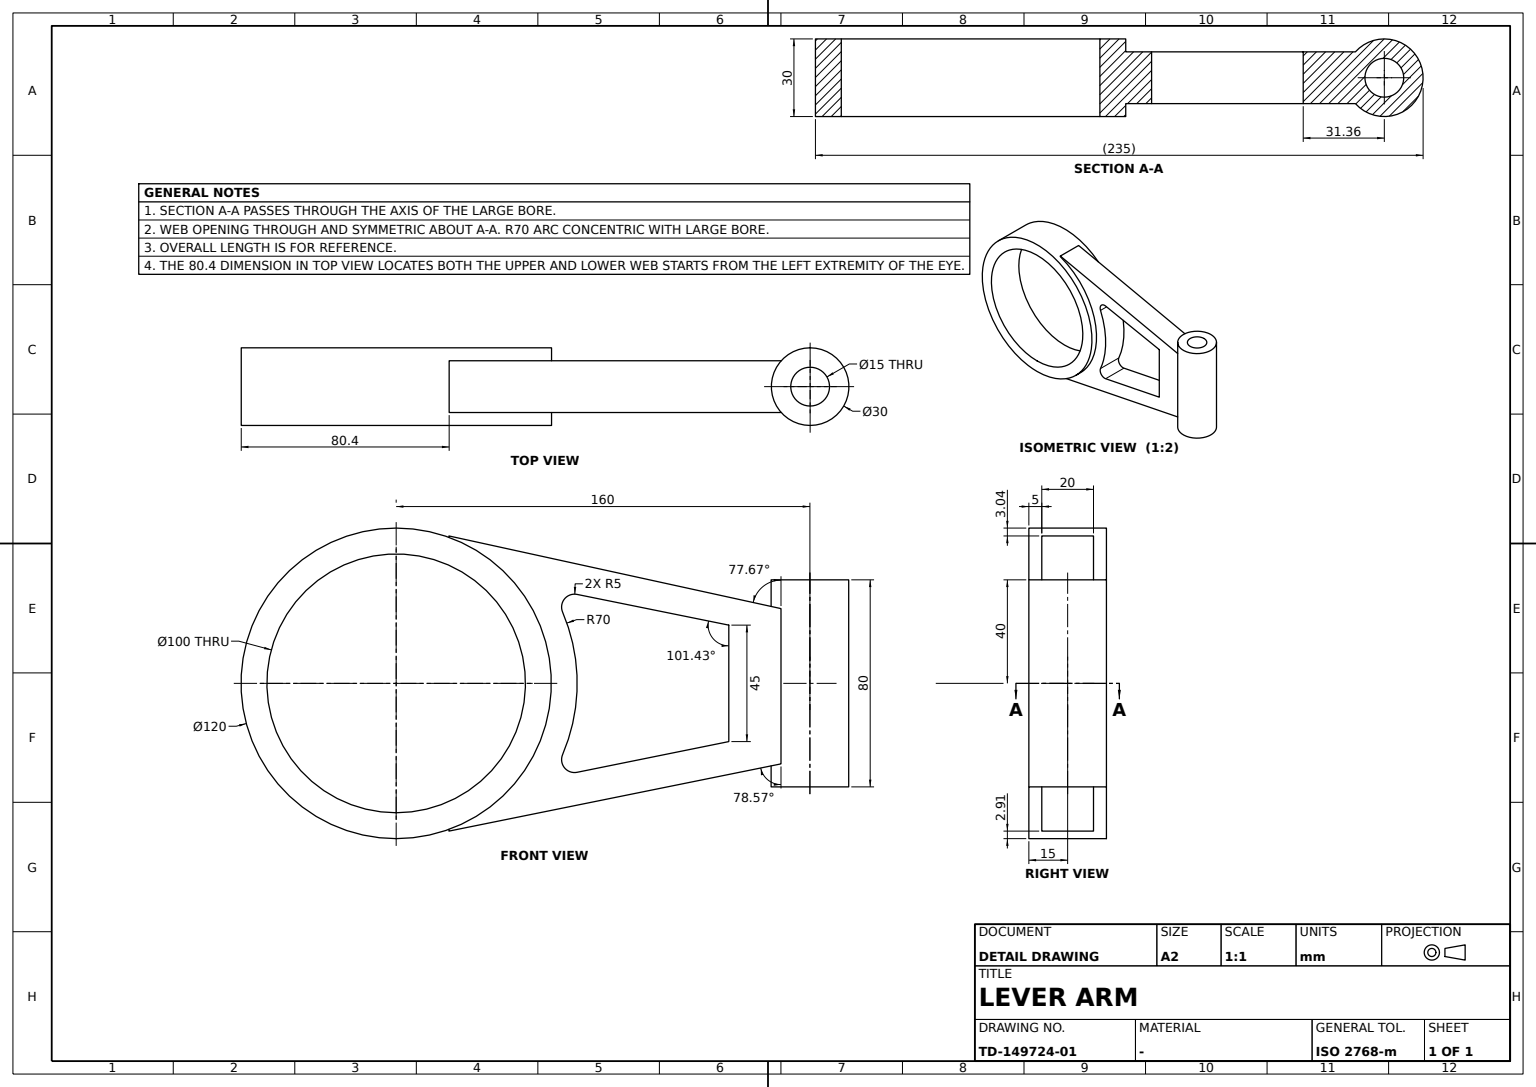
ISO-10303-21;
HEADER;
FILE_DESCRIPTION((''),'2;1');
FILE_NAME('','',(''),(''),'','','');
FILE_SCHEMA(('AUTOMOTIVE_DESIGN'));
ENDSEC;
DATA;
#1=APPLICATION_CONTEXT('');
#2=PRODUCT_CONTEXT('',#1,'mechanical');
#3=PRODUCT('','','',(#2));
#4=PRODUCT_DEFINITION_FORMATION('','',#3);
#5=PRODUCT_DEFINITION_CONTEXT('',#1,'design');
#6=PRODUCT_DEFINITION('','',#4,#5);
#7=PRODUCT_DEFINITION_SHAPE('','',#6);
#8=(LENGTH_UNIT()NAMED_UNIT(*)SI_UNIT(.MILLI.,.METRE.));
#9=(NAMED_UNIT(*)PLANE_ANGLE_UNIT()SI_UNIT($,.RADIAN.));
#10=(NAMED_UNIT(*)SI_UNIT($,.STERADIAN.)SOLID_ANGLE_UNIT());
#11=UNCERTAINTY_MEASURE_WITH_UNIT(LENGTH_MEASURE(0.005),#8,'distance_accuracy_value','');
#12=(GEOMETRIC_REPRESENTATION_CONTEXT(3)GLOBAL_UNCERTAINTY_ASSIGNED_CONTEXT((#11))GLOBAL_UNIT_ASSIGNED_CONTEXT((#8,#9,#10))REPRESENTATION_CONTEXT('',''));
#13=CARTESIAN_POINT('',(22.5,128.637224,-10.));
#14=VERTEX_POINT('',#13);
#15=CARTESIAN_POINT('',(34.367829,69.959986,-10.));
#16=VERTEX_POINT('',#15);
#17=DIRECTION('',(0.198241947,-0.980153116,0.));
#18=VECTOR('',#17,1000.);
#19=LINE('',#13,#18);
#20=EDGE_CURVE('',#14,#16,#19,.T.);
#21=ORIENTED_EDGE('',*,*,#20,.T.);
#22=CARTESIAN_POINT('',(34.367829,69.959986,10.));
#23=VERTEX_POINT('',#22);
#24=DIRECTION('',(0.,0.,1.));
#25=VECTOR('',#24,1000.);
#26=LINE('',#15,#25);
#27=EDGE_CURVE('',#23,#16,#26,.F.);
#28=ORIENTED_EDGE('',*,*,#27,.F.);
#29=CARTESIAN_POINT('',(22.5,128.637224,10.));
#30=VERTEX_POINT('',#29);
#31=CARTESIAN_POINT('',(42.646309,29.029308,10.));
#32=LINE('',#31,#18);
#33=EDGE_CURVE('',#30,#23,#32,.T.);
#34=ORIENTED_EDGE('',*,*,#33,.F.);
#35=DIRECTION('',(0.,0.,-1.));
#36=VECTOR('',#35,1000.);
#37=LINE('',#29,#36);
#38=EDGE_CURVE('',#30,#14,#37,.T.);
#39=ORIENTED_EDGE('',*,*,#38,.T.);
#40=EDGE_LOOP('',(#21,#28,#34,#39));
#41=FACE_BOUND('',#40,.T.);
#42=DIRECTION('',(0.980153116,0.198241947,0.));
#43=AXIS2_PLACEMENT_3D('',#29,#42,#17);
#44=PLANE('',#43);
#45=ADVANCED_FACE('',(#41),#44,.F.);
#46=CARTESIAN_POINT('',(56.424141,20.403831,-10.));
#47=VERTEX_POINT('',#46);
#48=CARTESIAN_POINT('',(56.424141,20.403831,10.));
#49=VERTEX_POINT('',#48);
#50=LINE('',#48,#25);
#51=EDGE_CURVE('',#47,#49,#50,.T.);
#52=ORIENTED_EDGE('',*,*,#51,.F.);
#53=CARTESIAN_POINT('',(57.088126,20.403831,-10.));
#54=VERTEX_POINT('',#53);
#55=CARTESIAN_POINT('',(0.,20.403831,-10.));
#56=DIRECTION('',(1.,0.,0.));
#57=VECTOR('',#56,1000.);
#58=LINE('',#55,#57);
#59=EDGE_CURVE('',#47,#54,#58,.T.);
#60=ORIENTED_EDGE('',*,*,#59,.T.);
#61=CARTESIAN_POINT('',(57.088126,20.403831,10.));
#62=VERTEX_POINT('',#61);
#63=LINE('',#61,#36);
#64=EDGE_CURVE('',#62,#54,#63,.T.);
#65=ORIENTED_EDGE('',*,*,#64,.F.);
#66=CARTESIAN_POINT('',(0.,20.403831,10.));
#67=LINE('',#66,#57);
#68=EDGE_CURVE('',#49,#62,#67,.T.);
#69=ORIENTED_EDGE('',*,*,#68,.F.);
#70=EDGE_LOOP('',(#52,#60,#65,#69));
#71=FACE_BOUND('',#70,.T.);
#72=DIRECTION('',(0.,-1.,0.));
#73=AXIS2_PLACEMENT_3D('',#66,#72,#35);
#74=PLANE('',#73);
#75=ADVANCED_FACE('',(#71),#74,.T.);
#76=CARTESIAN_POINT('',(-40.,160.,-15.));
#77=VERTEX_POINT('',#76);
#78=CARTESIAN_POINT('',(-40.,160.,0.));
#79=AXIS2_PLACEMENT_3D('',#78,#56,#35);
#80=CIRCLE('',#79,15.);
#81=EDGE_CURVE('',#77,#77,#80,.T.);
#82=ORIENTED_EDGE('',*,*,#81,.F.);
#83=EDGE_LOOP('',(#82));
#84=FACE_BOUND('',#83,.T.);
#85=CARTESIAN_POINT('',(-40.,160.,-7.5));
#86=VERTEX_POINT('',#85);
#87=CIRCLE('',#79,7.5);
#88=EDGE_CURVE('',#86,#86,#87,.T.);
#89=ORIENTED_EDGE('',*,*,#88,.T.);
#90=EDGE_LOOP('',(#89));
#91=FACE_BOUND('',#90,.T.);
#92=CARTESIAN_POINT('',(-40.,0.,0.));
#93=DIRECTION('',(0.,1.,0.));
#94=AXIS2_PLACEMENT_3D('',#92,#56,#93);
#95=PLANE('',#94);
#96=ADVANCED_FACE('',(#84,#91),#95,.F.);
#97=CARTESIAN_POINT('',(40.,160.,-7.5));
#98=VERTEX_POINT('',#97);
#99=CARTESIAN_POINT('',(40.,160.,0.));
#100=AXIS2_PLACEMENT_3D('',#99,#56,#35);
#101=CIRCLE('',#100,7.5);
#102=EDGE_CURVE('',#98,#98,#101,.T.);
#103=ORIENTED_EDGE('',*,*,#102,.T.);
#104=EDGE_LOOP('',(#103));
#105=FACE_BOUND('',#104,.T.);
#106=ORIENTED_EDGE('',*,*,#88,.F.);
#107=EDGE_LOOP('',(#106));
#108=FACE_BOUND('',#107,.T.);
#109=CARTESIAN_POINT('',(0.,160.,0.));
#110=AXIS2_PLACEMENT_3D('',#109,#56,#93);
#111=CYLINDRICAL_SURFACE('',#110,7.5);
#112=ADVANCED_FACE('',(#105,#108),#111,.F.);
#113=CARTESIAN_POINT('',(-34.367829,69.959986,10.));
#114=VERTEX_POINT('',#113);
#115=CARTESIAN_POINT('',(-34.367829,69.959986,-10.));
#116=VERTEX_POINT('',#115);
#117=LINE('',#115,#25);
#118=EDGE_CURVE('',#114,#116,#117,.F.);
#119=ORIENTED_EDGE('',*,*,#118,.F.);
#120=CARTESIAN_POINT('',(-27.502593,64.370858,10.));
#121=VERTEX_POINT('',#120);
#122=CARTESIAN_POINT('',(-29.467064,68.968777,10.));
#123=DIRECTION('',(-1.,0.,0.));
#124=AXIS2_PLACEMENT_3D('',#122,#35,#123);
#125=CIRCLE('',#124,5.);
#126=EDGE_CURVE('',#114,#121,#125,.F.);
#127=ORIENTED_EDGE('',*,*,#126,.T.);
#128=CARTESIAN_POINT('',(-27.502593,64.370858,-10.));
#129=VERTEX_POINT('',#128);
#130=CARTESIAN_POINT('',(-27.502593,64.370858,0.));
#131=LINE('',#130,#25);
#132=EDGE_CURVE('',#121,#129,#131,.F.);
#133=ORIENTED_EDGE('',*,*,#132,.T.);
#134=CARTESIAN_POINT('',(-29.467064,68.968777,-10.));
#135=AXIS2_PLACEMENT_3D('',#134,#24,#56);
#136=CIRCLE('',#135,5.);
#137=EDGE_CURVE('',#116,#129,#136,.T.);
#138=ORIENTED_EDGE('',*,*,#137,.F.);
#139=EDGE_LOOP('',(#119,#127,#133,#138));
#140=FACE_BOUND('',#139,.T.);
#141=CYLINDRICAL_SURFACE('',#135,5.);
#142=ADVANCED_FACE('',(#140),#141,.F.);
#143=CARTESIAN_POINT('',(50.,0.,-15.));
#144=VERTEX_POINT('',#143);
#145=CARTESIAN_POINT('',(0.,0.,-15.));
#146=AXIS2_PLACEMENT_3D('',#145,#24,#56);
#147=CIRCLE('',#146,50.);
#148=EDGE_CURVE('',#144,#144,#147,.T.);
#149=ORIENTED_EDGE('',*,*,#148,.T.);
#150=EDGE_LOOP('',(#149));
#151=FACE_BOUND('',#150,.T.);
#152=CARTESIAN_POINT('',(60.,0.,-15.));
#153=VERTEX_POINT('',#152);
#154=CIRCLE('',#146,60.);
#155=EDGE_CURVE('',#153,#153,#154,.T.);
#156=ORIENTED_EDGE('',*,*,#155,.F.);
#157=EDGE_LOOP('',(#156));
#158=FACE_BOUND('',#157,.T.);
#159=PLANE('',#146);
#160=ADVANCED_FACE('',(#151,#158),#159,.F.);
#161=CARTESIAN_POINT('',(-22.5,128.637224,10.));
#162=VERTEX_POINT('',#161);
#163=CARTESIAN_POINT('',(0.,128.637224,10.));
#164=LINE('',#163,#57);
#165=EDGE_CURVE('',#162,#30,#164,.T.);
#166=ORIENTED_EDGE('',*,*,#165,.T.);
#167=ORIENTED_EDGE('',*,*,#33,.T.);
#168=CARTESIAN_POINT('',(27.502593,64.370858,10.));
#169=VERTEX_POINT('',#168);
#170=CARTESIAN_POINT('',(29.467064,68.968777,10.));
#171=AXIS2_PLACEMENT_3D('',#170,#35,#123);
#172=CIRCLE('',#171,5.);
#173=EDGE_CURVE('',#169,#23,#172,.F.);
#174=ORIENTED_EDGE('',*,*,#173,.F.);
#175=CARTESIAN_POINT('',(0.,0.,10.));
#176=AXIS2_PLACEMENT_3D('',#175,#35,#123);
#177=CIRCLE('',#176,70.);
#178=EDGE_CURVE('',#169,#121,#177,.F.);
#179=ORIENTED_EDGE('',*,*,#178,.T.);
#180=ORIENTED_EDGE('',*,*,#126,.F.);
#181=CARTESIAN_POINT('',(-42.646309,29.029308,10.));
#182=DIRECTION('',(-0.198241947,-0.980153116,0.));
#183=VECTOR('',#182,1000.);
#184=LINE('',#181,#183);
#185=EDGE_CURVE('',#162,#114,#184,.T.);
#186=ORIENTED_EDGE('',*,*,#185,.F.);
#187=EDGE_LOOP('',(#166,#167,#174,#179,#180,#186));
#188=FACE_BOUND('',#187,.T.);
#189=CARTESIAN_POINT('',(31.115241,148.81966,10.));
#190=VERTEX_POINT('',#189);
#191=LINE('',#189,#18);
#192=EDGE_CURVE('',#190,#62,#191,.T.);
#193=ORIENTED_EDGE('',*,*,#192,.F.);
#194=CARTESIAN_POINT('',(-28.884759,148.81966,10.));
#195=VERTEX_POINT('',#194);
#196=LINE('',#194,#57);
#197=EDGE_CURVE('',#195,#190,#196,.T.);
#198=ORIENTED_EDGE('',*,*,#197,.F.);
#199=CARTESIAN_POINT('',(-56.956566,20.403831,10.));
#200=VERTEX_POINT('',#199);
#201=DIRECTION('',(-0.213557809,-0.976930429,0.));
#202=VECTOR('',#201,1000.);
#203=LINE('',#194,#202);
#204=EDGE_CURVE('',#195,#200,#203,.T.);
#205=ORIENTED_EDGE('',*,*,#204,.T.);
#206=CARTESIAN_POINT('',(-56.424141,20.403831,10.));
#207=VERTEX_POINT('',#206);
#208=EDGE_CURVE('',#200,#207,#67,.T.);
#209=ORIENTED_EDGE('',*,*,#208,.T.);
#210=CIRCLE('',#176,60.);
#211=EDGE_CURVE('',#207,#49,#210,.T.);
#212=ORIENTED_EDGE('',*,*,#211,.T.);
#213=ORIENTED_EDGE('',*,*,#68,.T.);
#214=EDGE_LOOP('',(#193,#198,#205,#209,#212,#213));
#215=FACE_BOUND('',#214,.T.);
#216=AXIS2_PLACEMENT_3D('',#66,#35,#93);
#217=PLANE('',#216);
#218=ADVANCED_FACE('',(#188,#215),#217,.F.);
#219=ORIENTED_EDGE('',*,*,#211,.F.);
#220=CARTESIAN_POINT('',(-56.424141,20.403831,-10.));
#221=VERTEX_POINT('',#220);
#222=LINE('',#206,#25);
#223=EDGE_CURVE('',#207,#221,#222,.F.);
#224=ORIENTED_EDGE('',*,*,#223,.T.);
#225=CARTESIAN_POINT('',(0.,0.,-10.));
#226=AXIS2_PLACEMENT_3D('',#225,#24,#56);
#227=CIRCLE('',#226,60.);
#228=EDGE_CURVE('',#47,#221,#227,.T.);
#229=ORIENTED_EDGE('',*,*,#228,.F.);
#230=ORIENTED_EDGE('',*,*,#51,.T.);
#231=EDGE_LOOP('',(#219,#224,#229,#230));
#232=FACE_BOUND('',#231,.T.);
#233=ORIENTED_EDGE('',*,*,#155,.T.);
#234=EDGE_LOOP('',(#233));
#235=FACE_BOUND('',#234,.T.);
#236=CARTESIAN_POINT('',(60.,0.,15.));
#237=VERTEX_POINT('',#236);
#238=CARTESIAN_POINT('',(0.,0.,15.));
#239=AXIS2_PLACEMENT_3D('',#238,#24,#56);
#240=CIRCLE('',#239,60.);
#241=EDGE_CURVE('',#237,#237,#240,.T.);
#242=ORIENTED_EDGE('',*,*,#241,.F.);
#243=EDGE_LOOP('',(#242));
#244=FACE_BOUND('',#243,.T.);
#245=CARTESIAN_POINT('',(0.,0.,0.));
#246=AXIS2_PLACEMENT_3D('',#245,#24,#56);
#247=CYLINDRICAL_SURFACE('',#246,60.);
#248=ADVANCED_FACE('',(#232,#235,#244),#247,.T.);
#249=CARTESIAN_POINT('',(50.,0.,15.));
#250=VERTEX_POINT('',#249);
#251=CIRCLE('',#239,50.);
#252=EDGE_CURVE('',#250,#250,#251,.T.);
#253=ORIENTED_EDGE('',*,*,#252,.T.);
#254=EDGE_LOOP('',(#253));
#255=FACE_BOUND('',#254,.T.);
#256=ORIENTED_EDGE('',*,*,#148,.F.);
#257=EDGE_LOOP('',(#256));
#258=FACE_BOUND('',#257,.T.);
#259=CYLINDRICAL_SURFACE('',#246,50.);
#260=ADVANCED_FACE('',(#255,#258),#259,.F.);
#261=ORIENTED_EDGE('',*,*,#178,.F.);
#262=CARTESIAN_POINT('',(27.502593,64.370858,-10.));
#263=VERTEX_POINT('',#262);
#264=CARTESIAN_POINT('',(27.502593,64.370858,0.));
#265=LINE('',#264,#25);
#266=EDGE_CURVE('',#169,#263,#265,.F.);
#267=ORIENTED_EDGE('',*,*,#266,.T.);
#268=CIRCLE('',#226,70.);
#269=EDGE_CURVE('',#263,#129,#268,.T.);
#270=ORIENTED_EDGE('',*,*,#269,.T.);
#271=ORIENTED_EDGE('',*,*,#132,.F.);
#272=EDGE_LOOP('',(#261,#267,#270,#271));
#273=FACE_BOUND('',#272,.T.);
#274=CYLINDRICAL_SURFACE('',#226,70.);
#275=ADVANCED_FACE('',(#273),#274,.T.);
#276=CARTESIAN_POINT('',(-22.5,128.637224,-10.));
#277=VERTEX_POINT('',#276);
#278=LINE('',#276,#57);
#279=EDGE_CURVE('',#277,#14,#278,.T.);
#280=ORIENTED_EDGE('',*,*,#279,.T.);
#281=ORIENTED_EDGE('',*,*,#38,.F.);
#282=ORIENTED_EDGE('',*,*,#165,.F.);
#283=LINE('',#161,#36);
#284=EDGE_CURVE('',#162,#277,#283,.T.);
#285=ORIENTED_EDGE('',*,*,#284,.T.);
#286=EDGE_LOOP('',(#280,#281,#282,#285));
#287=FACE_BOUND('',#286,.T.);
#288=AXIS2_PLACEMENT_3D('',#161,#93,#56);
#289=PLANE('',#288);
#290=ADVANCED_FACE('',(#287),#289,.F.);
#291=ORIENTED_EDGE('',*,*,#185,.T.);
#292=ORIENTED_EDGE('',*,*,#118,.T.);
#293=LINE('',#276,#183);
#294=EDGE_CURVE('',#277,#116,#293,.T.);
#295=ORIENTED_EDGE('',*,*,#294,.F.);
#296=ORIENTED_EDGE('',*,*,#284,.F.);
#297=EDGE_LOOP('',(#291,#292,#295,#296));
#298=FACE_BOUND('',#297,.T.);
#299=DIRECTION('',(0.980153116,-0.198241947,0.));
#300=AXIS2_PLACEMENT_3D('',#161,#299,#182);
#301=PLANE('',#300);
#302=ADVANCED_FACE('',(#298),#301,.T.);
#303=CARTESIAN_POINT('',(31.115241,148.81966,-10.));
#304=VERTEX_POINT('',#303);
#305=CARTESIAN_POINT('',(29.892417,154.865584,-10.));
#306=LINE('',#305,#18);
#307=EDGE_CURVE('',#304,#54,#306,.T.);
#308=ORIENTED_EDGE('',*,*,#307,.F.);
#309=CARTESIAN_POINT('',(28.85395,160.,0.));
#310=DIRECTION('',(-0.980153116,-0.198241947,0.));
#311=AXIS2_PLACEMENT_3D('',#309,#310,#17);
#312=ELLIPSE('',#311,15.303731,15.);
#313=EDGE_CURVE('',#304,#190,#312,.T.);
#314=ORIENTED_EDGE('',*,*,#313,.T.);
#315=ORIENTED_EDGE('',*,*,#192,.T.);
#316=ORIENTED_EDGE('',*,*,#64,.T.);
#317=EDGE_LOOP('',(#308,#314,#315,#316));
#318=FACE_BOUND('',#317,.T.);
#319=CARTESIAN_POINT('',(31.115241,148.81966,0.));
#320=AXIS2_PLACEMENT_3D('',#319,#310,#17);
#321=PLANE('',#320);
#322=ADVANCED_FACE('',(#318),#321,.F.);
#323=ORIENTED_EDGE('',*,*,#223,.F.);
#324=ORIENTED_EDGE('',*,*,#208,.F.);
#325=CARTESIAN_POINT('',(-56.956566,20.403831,-10.));
#326=VERTEX_POINT('',#325);
#327=LINE('',#199,#36);
#328=EDGE_CURVE('',#200,#326,#327,.T.);
#329=ORIENTED_EDGE('',*,*,#328,.T.);
#330=EDGE_CURVE('',#326,#221,#58,.T.);
#331=ORIENTED_EDGE('',*,*,#330,.T.);
#332=EDGE_LOOP('',(#323,#324,#329,#331));
#333=FACE_BOUND('',#332,.T.);
#334=ADVANCED_FACE('',(#333),#74,.T.);
#335=ORIENTED_EDGE('',*,*,#81,.T.);
#336=EDGE_LOOP('',(#335));
#337=FACE_BOUND('',#336,.T.);
#338=CARTESIAN_POINT('',(40.,160.,-15.));
#339=VERTEX_POINT('',#338);
#340=CIRCLE('',#100,15.);
#341=EDGE_CURVE('',#339,#339,#340,.T.);
#342=ORIENTED_EDGE('',*,*,#341,.F.);
#343=EDGE_LOOP('',(#342));
#344=FACE_BOUND('',#343,.T.);
#345=ORIENTED_EDGE('',*,*,#197,.T.);
#346=ORIENTED_EDGE('',*,*,#313,.F.);
#347=CARTESIAN_POINT('',(-28.884759,148.81966,-10.));
#348=VERTEX_POINT('',#347);
#349=LINE('',#347,#57);
#350=EDGE_CURVE('',#348,#304,#349,.T.);
#351=ORIENTED_EDGE('',*,*,#350,.F.);
#352=CARTESIAN_POINT('',(-26.440727,160.,0.));
#353=DIRECTION('',(-0.976930429,0.213557809,0.));
#354=DIRECTION('',(0.213557809,0.976930429,0.));
#355=AXIS2_PLACEMENT_3D('',#352,#353,#354);
#356=ELLIPSE('',#355,15.354215,15.);
#357=EDGE_CURVE('',#348,#195,#356,.T.);
#358=ORIENTED_EDGE('',*,*,#357,.T.);
#359=EDGE_LOOP('',(#345,#346,#351,#358));
#360=FACE_BOUND('',#359,.T.);
#361=CYLINDRICAL_SURFACE('',#110,15.);
#362=ADVANCED_FACE('',(#337,#344,#360),#361,.T.);
#363=ORIENTED_EDGE('',*,*,#341,.T.);
#364=EDGE_LOOP('',(#363));
#365=FACE_BOUND('',#364,.T.);
#366=ORIENTED_EDGE('',*,*,#102,.F.);
#367=EDGE_LOOP('',(#366));
#368=FACE_BOUND('',#367,.T.);
#369=CARTESIAN_POINT('',(40.,0.,0.));
#370=AXIS2_PLACEMENT_3D('',#369,#56,#93);
#371=PLANE('',#370);
#372=ADVANCED_FACE('',(#365,#368),#371,.T.);
#373=ORIENTED_EDGE('',*,*,#173,.T.);
#374=ORIENTED_EDGE('',*,*,#27,.T.);
#375=CARTESIAN_POINT('',(29.467064,68.968777,-10.));
#376=AXIS2_PLACEMENT_3D('',#375,#24,#56);
#377=CIRCLE('',#376,5.);
#378=EDGE_CURVE('',#263,#16,#377,.T.);
#379=ORIENTED_EDGE('',*,*,#378,.F.);
#380=ORIENTED_EDGE('',*,*,#266,.F.);
#381=EDGE_LOOP('',(#373,#374,#379,#380));
#382=FACE_BOUND('',#381,.T.);
#383=CYLINDRICAL_SURFACE('',#376,5.);
#384=ADVANCED_FACE('',(#382),#383,.F.);
#385=ORIENTED_EDGE('',*,*,#328,.F.);
#386=ORIENTED_EDGE('',*,*,#204,.F.);
#387=ORIENTED_EDGE('',*,*,#357,.F.);
#388=CARTESIAN_POINT('',(-27.567413,154.84592,-10.));
#389=LINE('',#388,#202);
#390=EDGE_CURVE('',#348,#326,#389,.T.);
#391=ORIENTED_EDGE('',*,*,#390,.T.);
#392=EDGE_LOOP('',(#385,#386,#387,#391));
#393=FACE_BOUND('',#392,.T.);
#394=CARTESIAN_POINT('',(-28.884759,148.81966,0.));
#395=AXIS2_PLACEMENT_3D('',#394,#353,#201);
#396=PLANE('',#395);
#397=ADVANCED_FACE('',(#393),#396,.T.);
#398=ORIENTED_EDGE('',*,*,#307,.T.);
#399=ORIENTED_EDGE('',*,*,#59,.F.);
#400=ORIENTED_EDGE('',*,*,#228,.T.);
#401=ORIENTED_EDGE('',*,*,#330,.F.);
#402=ORIENTED_EDGE('',*,*,#390,.F.);
#403=ORIENTED_EDGE('',*,*,#350,.T.);
#404=EDGE_LOOP('',(#398,#399,#400,#401,#402,#403));
#405=FACE_BOUND('',#404,.T.);
#406=ORIENTED_EDGE('',*,*,#279,.F.);
#407=ORIENTED_EDGE('',*,*,#294,.T.);
#408=ORIENTED_EDGE('',*,*,#137,.T.);
#409=ORIENTED_EDGE('',*,*,#269,.F.);
#410=ORIENTED_EDGE('',*,*,#378,.T.);
#411=ORIENTED_EDGE('',*,*,#20,.F.);
#412=EDGE_LOOP('',(#406,#407,#408,#409,#410,#411));
#413=FACE_BOUND('',#412,.T.);
#414=CARTESIAN_POINT('',(0.,148.81966,-10.));
#415=AXIS2_PLACEMENT_3D('',#414,#24,#72);
#416=PLANE('',#415);
#417=ADVANCED_FACE('',(#405,#413),#416,.F.);
#418=ORIENTED_EDGE('',*,*,#252,.F.);
#419=EDGE_LOOP('',(#418));
#420=FACE_BOUND('',#419,.T.);
#421=ORIENTED_EDGE('',*,*,#241,.T.);
#422=EDGE_LOOP('',(#421));
#423=FACE_BOUND('',#422,.T.);
#424=PLANE('',#239);
#425=ADVANCED_FACE('',(#420,#423),#424,.T.);
#426=CLOSED_SHELL('',(#45,#75,#96,#112,#142,#160,#218,#248,#260,#275,#290,#302,#322,#334,#362,#372,#384,#397,#417,#425));
#427=MANIFOLD_SOLID_BREP('',#426);
#428=ADVANCED_BREP_SHAPE_REPRESENTATION('',(#427),#12);
#429=SHAPE_DEFINITION_REPRESENTATION(#7,#428);
ENDSEC;
END-ISO-10303-21;
